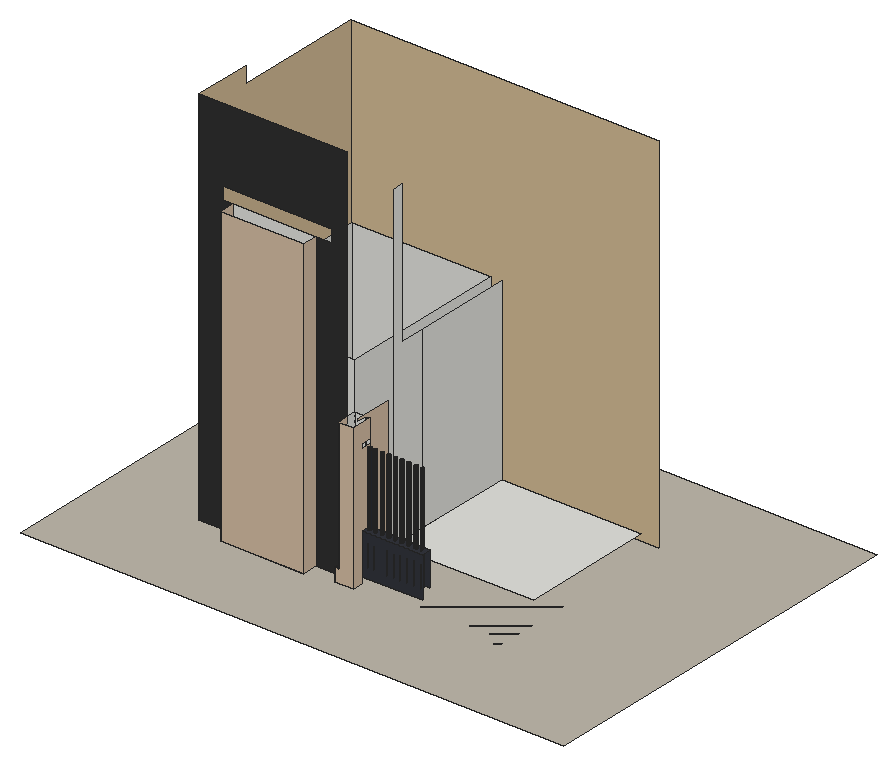
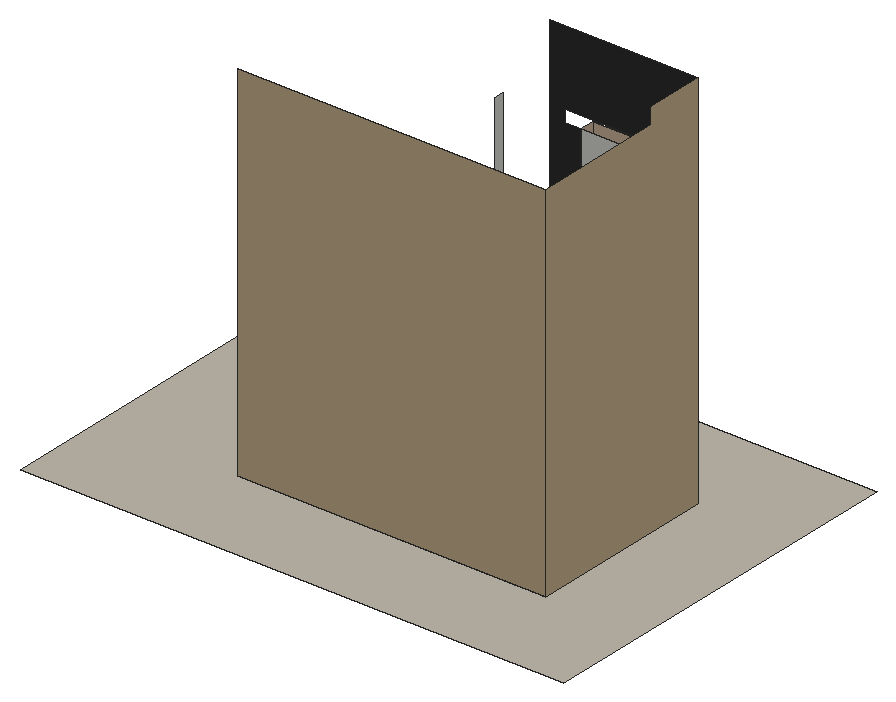
# SketchUp Ruby script. Lengths in inches.
U = 1.inch
M = Sketchup.active_model
def pt(a) = Geom::Point3d.new(a.map { |v| v * U })
def face(e, loops, mat)
  f = e.add_face(loops[0].map { |a| pt(a) })
  loops[1..].each { |l| e.add_face(l.map { |a| pt(a) }).erase! }
  f.material = f.back_material = mat if mat
  f
end
# faces: each face lists its corners as indices into pts; further lists are holes
def faces(e, pts, list, mat = nil) = list.each { |f| face(e, (f[0].is_a?(Array) ? f : [f]).map { |l| l.map { |i| pts[i] } }, mat) }
# xy, xz, yz: faces in a plane at the given z, y or x. An outline is a flat list of corners, or four numbers for a rectangle; further outlines are holes
def ring(l) = l.size == 4 ? [[l[0], l[1]], [l[2], l[1]], [l[2], l[3]], [l[0], l[3]]] : l.each_slice(2).to_a
def flat(e, list, mat, &to3) = list.each { |f| face(e, (f[0].is_a?(Array) ? f : [f]).map { |l| ring(l).map { |u, v| to3.(u, v) } }, mat) }
def xy(e, z, list, mat = nil) = flat(e, list, mat) { |x, y| [x, y, z] }
def xz(e, y, list, mat = nil) = flat(e, list, mat) { |x, z| [x, y, z] }
def yz(e, x, list, mat = nil) = flat(e, list, mat) { |y, z| [x, y, z] }
def lines(e, pts, list) = list.each { |a, b| e.add_line(pt(pts[a]), pt(pts[b])) }
# prism: a flat outline (further loops are holes) pulled along v
def prism(e, loops, v, mat = nil)
  f = face(e, loops, mat); d = Geom::Vector3d.new(v.map { |x| x * U })
  f.pushpull(f.normal.samedirection?(d) ? d.length : -d.length)
end
def box(e, o, s, mat = nil) = prism(e, [[o, [o[0] + s[0], o[1], o[2]], [o[0] + s[0], o[1] + s[1], o[2]], [o[0], o[1] + s[1], o[2]]]], [0, 0, s[2]], mat)
def at(x, y, z, deg = 0) = Geom::Transformation.translation(pt([x, y, z])) * Geom::Transformation.rotation(ORIGIN, Z_AXIS, deg.degrees)
def axes(o, x, y, z) = Geom::Transformation.new([*x, 0, *y, 0, *z, 0, *pt(o).to_a, 1])
def part(name) = M.definitions.add(name)
# library, detail: a bought-in or finely detailed component or shape, given as its bounding box
def library(name, o, s) = part(name).tap { |d| box(d.entities, o, s) }
def detail(e, o, s) = box(e.add_group.entities, o, s)
def put(e, d, t, mat = nil) = e.add_instance(d, t).tap { |i| i.material = mat if mat }
def group(e, t, mat = nil) = e.add_group.tap { |g| g.transformation = t; g.material = mat if mat }.entities
root = M.entities
M.materials.add("[Cinder Block]").color = [191, 184, 171]
M.materials.add("[Concrete Block 8x8 Gray]").color = [48, 48, 47]
M.materials.add("[Formica Beige]").color = [211, 187, 149]
M.materials.add("[Formica Laminate Dark]").color = [50, 53, 60]
M.materials.add("[Formica Laminate Light]").color = [213, 189, 164]
xy(root,0,[[87.96,59.04,144.31,69.35],[162.85,61.98,162.85,69.35,65.24,69.35,65.24,197.12,273.31,197.12,273.31,61.98,261.51,61.98,261.51,69.35,175.36,69.35,175.36,61.98]])
xy(root,0,[[[0,0,367.4375,263.4375],[87.96,59.04,144.31,69.35]]],"[Cinder Block]")
xy(root,9,[[177.5,71.93,177.24,71.96,177,72.0625,176.79,72.22,176.63,72.43,176.53,72.67,176.5,72.93,176.53,73.1875,176.63,73.43,176.79,73.63,177,73.79,177.24,73.89,177.5,73.93,177.76,73.89,178,73.79,178.21,73.63,178.37,73.43,178.46,73.1875,178.5,72.93,178.46,72.67,178.37,72.43,178.21,72.22,178,72.0625,177.76,71.96],[181.5,71.93,181.24,71.96,181,72.0625,180.79,72.22,180.63,72.43,180.53,72.67,180.5,72.93,180.53,73.1875,180.63,73.43,180.79,73.63,181,73.79,181.24,73.89,181.5,73.93,181.76,73.89,182,73.79,182.21,73.63,182.37,73.43,182.46,73.1875,182.5,72.93,182.46,72.67,182.37,72.43,182.21,72.22,182,72.0625,181.76,71.96],[186.1875,71.93,185.93,71.96,185.6875,72.0625,185.48,72.22,185.32,72.43,185.22,72.67,185.1875,72.93,185.22,73.1875,185.32,73.43,185.48,73.63,185.6875,73.79,185.93,73.89,186.1875,73.93,186.45,73.89,186.6875,73.79,186.89,73.63,187.05,73.43,187.15,73.1875,187.1875,72.93,187.15,72.67,187.05,72.43,186.89,72.22,186.6875,72.0625,186.45,71.96],[190.75,71.93,190.49,71.96,190.25,72.0625,190.04,72.22,189.88,72.43,189.78,72.67,189.75,72.93,189.78,73.1875,189.88,73.43,190.04,73.63,190.25,73.79,190.49,73.89,190.75,73.93,191.01,73.89,191.25,73.79,191.46,73.63,191.62,73.43,191.71,73.1875,191.75,72.93,191.71,72.67,191.62,72.43,191.46,72.22,191.25,72.0625,191.01,71.96],[195,71.93,194.74,71.96,194.5,72.0625,194.29,72.22,194.13,72.43,194.03,72.67,194,72.93,194.03,73.1875,194.13,73.43,194.29,73.63,194.5,73.79,194.74,73.89,195,73.93,195.26,73.89,195.5,73.79,195.71,73.63,195.87,73.43,195.96,73.1875,196,72.93,195.96,72.67,195.87,72.43,195.71,72.22,195.5,72.0625,195.26,71.96],
  [199.4375,71.93,199.18,71.96,198.9375,72.0625,198.73,72.22,198.57,72.43,198.47,72.67,198.4375,72.93,198.47,73.1875,198.57,73.43,198.73,73.63,198.9375,73.79,199.18,73.89,199.4375,73.93,199.7,73.89,199.9375,73.79,200.14,73.63,200.3,73.43,200.4,73.1875,200.4375,72.93,200.4,72.67,200.3,72.43,200.14,72.22,199.9375,72.0625,199.7,71.96],[204,71.93,203.74,71.96,203.5,72.0625,203.29,72.22,203.13,72.43,203.03,72.67,203,72.93,203.03,73.1875,203.13,73.43,203.29,73.63,203.5,73.79,203.74,73.89,204,73.93,204.26,73.89,204.5,73.79,204.71,73.63,204.87,73.43,204.96,73.1875,205,72.93,204.96,72.67,204.87,72.43,204.71,72.22,204.5,72.0625,204.26,71.96],[209.0625,71.93,208.8,71.96,208.5625,72.0625,208.35,72.22,208.2,72.43,208.1,72.67,208.0625,72.93,208.1,73.1875,208.2,73.43,208.35,73.63,208.5625,73.79,208.8,73.89,209.0625,73.93,209.32,73.89,209.5625,73.79,209.77,73.63,209.93,73.43,210.03,73.1875,210.0625,72.93,210.03,72.67,209.93,72.43,209.77,72.22,209.5625,72.0625,209.32,71.96],[71.76,75.87,165.35,190.6],[172.48,99.67,266.79,190.6]])
xy(root,9,[[162.85,61.98,165.35,69.35]],"[Formica Laminate Light]")
xy(root,32.25,[[[175.36,69.35,216.21,75.87],[177.5,71.93,177.24,71.96,177,72.0625,176.79,72.22,176.63,72.43,176.53,72.67,176.5,72.93,176.53,73.1875,176.63,73.43,176.79,73.63,177,73.79,177.24,73.89,177.5,73.93,177.76,73.89,178,73.79,178.21,73.63,178.37,73.43,178.46,73.1875,178.5,72.93,178.46,72.67,178.37,72.43,178.21,72.22,178,72.0625,177.76,71.96],[213.5,71.93,213.24,71.96,213,72.0625,212.79,72.22,212.63,72.43,212.53,72.67,212.5,72.93,212.53,73.1875,212.63,73.43,212.79,73.63,213,73.79,213.24,73.89,213.5,73.93,213.76,73.89,214,73.79,214.21,73.63,214.37,73.43,214.46,73.1875,214.5,72.93,214.46,72.67,214.37,72.43,214.21,72.22,214,72.0625,213.76,71.96],[181.5,71.93,181.24,71.96,181,72.0625,180.79,72.22,180.63,72.43,180.53,72.67,180.5,72.93,180.53,73.1875,180.63,73.43,180.79,73.63,181,73.79,181.24,73.89,181.5,73.93,181.76,73.89,182,73.79,182.21,73.63,182.37,73.43,182.46,73.1875,182.5,72.93,182.46,72.67,182.37,72.43,182.21,72.22,182,72.0625,181.76,71.96],[209.0625,71.93,208.8,71.96,208.5625,72.0625,208.35,72.22,208.2,72.43,208.1,72.67,208.0625,72.93,208.1,73.1875,208.2,73.43,208.35,73.63,208.5625,73.79,208.8,73.89,209.0625,73.93,209.32,73.89,209.5625,73.79,209.77,73.63,209.93,73.43,210.03,73.1875,210.0625,72.93,210.03,72.67,209.93,72.43,209.77,72.22,209.5625,72.0625,209.32,71.96],[186.1875,71.93,185.93,71.96,185.6875,72.0625,185.48,72.22,185.32,72.43,185.22,72.67,185.1875,72.93,185.22,73.1875,185.32,73.43,185.48,73.63,185.6875,73.79,185.93,73.89,186.1875,73.93,186.45,73.89,186.6875,73.79,186.89,73.63,187.05,73.43,187.15,73.1875,187.1875,72.93,187.15,72.67,187.05,72.43,186.89,72.22,186.6875,72.0625,186.45,71.96],[204,71.93,203.74,71.96,203.5,72.0625,203.29,72.22,203.13,72.43,203.03,72.67,203,72.93,203.03,73.1875,203.13,73.43,203.29,73.63,203.5,73.79,203.74,73.89,204,73.93,204.26,73.89,204.5,73.79,204.71,73.63,204.87,73.43,204.96,73.1875,205,72.93,204.96,72.67,204.87,72.43,204.71,72.22,204.5,72.0625,204.26,71.96],[190.75,71.93,190.49,71.96,190.25,72.0625,190.04,72.22,189.88,72.43,189.78,72.67,189.75,72.93,189.78,73.1875,189.88,73.43,190.04,73.63,190.25,73.79,190.49,73.89,190.75,73.93,191.01,73.89,191.25,73.79,191.46,73.63,191.62,73.43,191.71,73.1875,191.75,72.93,191.71,72.67,191.62,72.43,191.46,72.22,191.25,72.0625,191.01,71.96],[199.4375,71.93,199.18,71.96,198.9375,72.0625,198.73,72.22,198.57,72.43,198.47,72.67,198.4375,72.93,198.47,73.1875,198.57,73.43,198.73,73.63,198.9375,73.79,199.18,73.89,199.4375,73.93,199.7,73.89,199.9375,73.79,200.14,73.63,200.3,73.43,200.4,73.1875,200.4375,72.93,200.4,72.67,200.3,72.43,200.14,72.22,199.9375,72.0625,199.7,71.96],[195,71.93,194.74,71.96,194.5,72.0625,194.29,72.22,194.13,72.43,194.03,72.67,194,72.93,194.03,73.1875,194.13,73.43,194.29,73.63,194.5,73.79,194.74,73.89,195,73.93,195.26,73.89,195.5,73.79,195.71,73.63,195.87,73.43,195.96,73.1875,196,72.93,195.96,72.67,195.87,72.43,195.71,72.22,195.5,72.0625,195.26,71.96]]],"[Formica Laminate Dark]")
xz(root,59.04,[[87.96,0,144.31,199.15]],"[Formica Laminate Light]")
xz(root,61.98,[[162.85,0,175.36,0,175.36,97.5,165.35,97.5,165.35,9,162.85,9]],"[Formica Laminate Light]")
xz(root,69.35,[[87.96,0,144.31,199.15]])
xz(root,69.35,[[65.24,0,87.96,0,87.96,199.15,81.08,199.15,81.08,207.68,154.75,207.68,154.75,199.15,144.31,199.15,144.31,0,162.85,0,162.85,9,165.35,9,165.35,257.76,65.24,257.76]],"[Concrete Block 8x8 Gray]")
xz(root,69.35,[[175.36,4.5,216.21,32.25]],"[Formica Laminate Dark]")
xz(root,75.87,[[71.76,9,165.35,129],[165.35,9,172.48,97.5],[172.48,9,175.36,97.5]])
xz(root,75.87,[[175.36,9,216.21,32.25]],"[Formica Laminate Dark]")
xz(root,190.6,[[71.76,9,165.35,129]])
xz(root,197.12,[[65.24,0,273.31,246.5]],"[Formica Beige]")
yz(root,65.24,[[69.35,0,69.35,257.76,108.74,257.76,108.74,246.5,197.12,246.5,197.12,0]],"[Formica Beige]")
yz(root,71.76,[[75.87,9,190.6,129]])
yz(root,87.96,[[59.04,0,69.35,199.15]],"[Formica Laminate Light]")
yz(root,144.31,[[59.04,0,69.35,199.15]],"[Formica Laminate Light]")
yz(root,162.85,[[61.98,0,69.35,9]],"[Formica Laminate Light]")
yz(root,165.35,[[69.35,9,75.87,97.5],[75.87,9,190.6,129]])
yz(root,165.35,[[61.98,9,69.35,97.5]],"[Formica Laminate Light]")
yz(root,172.48,[[99.67,9,123.48,9,123.48,129,106.73,129,106.73,224.375,99.67,224.375],[123.48,9,190.6,129]])
yz(root,172.48,[[75.87,9,94.48,9,94.48,98.95,69.35,98.95,69.35,97.5,75.87,97.5]],"[Formica Laminate Light]")
yz(root,175.36,[[61.98,0,69.35,0,69.35,32.25,75.87,32.25,75.87,81.84,69.35,81.84,69.35,84.9,75.87,84.9,75.87,97.5,61.98,97.5]],"[Formica Laminate Light]")
p = [[177.24,71.96,9],[177.5,71.93,9],[177.5,71.93,32.25],[177.24,71.96,32.25],[177.76,71.96,9],[177.76,71.96,32.25],
  [181.24,71.96,9],[181.5,71.93,9],[181.5,71.93,32.25],[181.24,71.96,32.25],[181.76,71.96,9],[181.76,71.96,32.25],
  [185.93,71.96,9],[186.1875,71.93,9],[186.1875,71.93,32.25],[185.93,71.96,32.25],[186.45,71.96,9],[186.45,71.96,32.25],
  [190.49,71.96,9],[190.75,71.93,9],[190.75,71.93,32.25],[190.49,71.96,32.25],[191.01,71.96,9],[191.01,71.96,32.25],
  [194.74,71.96,9],[195,71.93,9],[195,71.93,32.25],[194.74,71.96,32.25],[195.26,71.96,9],[195.26,71.96,32.25],
  [199.18,71.96,9],[199.4375,71.93,9],[199.4375,71.93,32.25],[199.18,71.96,32.25],[199.7,71.96,9],[199.7,71.96,32.25],
  [203.74,71.96,9],[204,71.93,9],[204,71.93,32.25],[203.74,71.96,32.25],[204.26,71.96,9],[204.26,71.96,32.25],
  [208.8,71.96,9],[209.0625,71.93,9],[209.0625,71.93,32.25],[208.8,71.96,32.25],[209.32,71.96,9],[209.32,71.96,32.25],
  [213.24,71.96,9],[213.5,71.93,9],[213.5,71.93,32.25],[213.24,71.96,32.25],[177,72.0625,9],[177,72.0625,32.25],
  [178,72.0625,9],[178,72.0625,32.25],[181,72.0625,9],[181,72.0625,32.25],[182,72.0625,9],[182,72.0625,32.25],
  [185.6875,72.0625,9],[185.6875,72.0625,32.25],[186.6875,72.0625,9],[186.6875,72.0625,32.25],[190.25,72.0625,9],[190.25,72.0625,32.25],
  [191.25,72.0625,9],[191.25,72.0625,32.25],[194.5,72.0625,9],[194.5,72.0625,32.25],[195.5,72.0625,9],[195.5,72.0625,32.25],
  [198.9375,72.0625,9],[198.9375,72.0625,32.25],[199.9375,72.0625,9],[199.9375,72.0625,32.25],[203.5,72.0625,9],[203.5,72.0625,32.25],
  [204.5,72.0625,9],[204.5,72.0625,32.25],[208.5625,72.0625,9],[208.5625,72.0625,32.25],[209.5625,72.0625,9],[209.5625,72.0625,32.25],
  [213,72.0625,9],[213,72.0625,32.25],[176.79,72.22,9],[176.79,72.22,32.25],[178.21,72.22,9],[178.21,72.22,32.25],
  [180.79,72.22,9],[180.79,72.22,32.25],[182.21,72.22,9],[182.21,72.22,32.25],[185.48,72.22,9],[185.48,72.22,32.25],
  [186.89,72.22,9],[186.89,72.22,32.25],[190.04,72.22,9],[190.04,72.22,32.25],[191.46,72.22,9],[191.46,72.22,32.25],
  [194.29,72.22,9],[194.29,72.22,32.25],[195.71,72.22,9],[195.71,72.22,32.25],[198.73,72.22,9],[198.73,72.22,32.25],
  [200.14,72.22,9],[200.14,72.22,32.25],[203.29,72.22,9],[203.29,72.22,32.25],[204.71,72.22,9],[204.71,72.22,32.25],
  [208.35,72.22,9],[208.35,72.22,32.25],[209.77,72.22,9],[209.77,72.22,32.25],[212.79,72.22,9],[212.79,72.22,32.25],
  [176.63,72.43,9],[176.63,72.43,32.25],[178.37,72.43,9],[178.37,72.43,32.25],[180.63,72.43,9],[180.63,72.43,32.25],
  [182.37,72.43,9],[182.37,72.43,32.25],[185.32,72.43,9],[185.32,72.43,32.25],[187.05,72.43,9],[187.05,72.43,32.25],
  [189.88,72.43,9],[189.88,72.43,32.25],[191.62,72.43,9],[191.62,72.43,32.25],[194.13,72.43,9],[194.13,72.43,32.25],
  [195.87,72.43,9],[195.87,72.43,32.25],[198.57,72.43,9],[198.57,72.43,32.25],[200.3,72.43,9],[200.3,72.43,32.25],
  [203.13,72.43,9],[203.13,72.43,32.25],[204.87,72.43,9],[204.87,72.43,32.25],[208.2,72.43,9],[208.2,72.43,32.25],
  [209.93,72.43,9],[209.93,72.43,32.25],[212.63,72.43,9],[212.63,72.43,32.25],[176.53,72.67,9],[176.53,72.67,32.25],
  [178.46,72.67,9],[178.46,72.67,32.25],[180.53,72.67,9],[180.53,72.67,32.25],[182.46,72.67,9],[182.46,72.67,32.25],
  [185.22,72.67,9],[185.22,72.67,32.25],[187.15,72.67,9],[187.15,72.67,32.25],[189.78,72.67,9],[189.78,72.67,32.25],
  [191.71,72.67,9],[191.71,72.67,32.25],[194.03,72.67,9],[194.03,72.67,32.25],[195.96,72.67,9],[195.96,72.67,32.25],
  [198.47,72.67,9],[198.47,72.67,32.25],[200.4,72.67,9],[200.4,72.67,32.25],[203.03,72.67,9],[203.03,72.67,32.25],
  [204.96,72.67,9],[204.96,72.67,32.25],[208.1,72.67,9],[208.1,72.67,32.25],[210.03,72.67,9],[210.03,72.67,32.25],
  [212.53,72.67,9],[212.53,72.67,32.25],[176.5,72.93,9],[176.5,72.93,32.25],[178.5,72.93,9],[178.5,72.93,32.25],
  [180.5,72.93,9],[180.5,72.93,32.25],[182.5,72.93,9],[182.5,72.93,32.25],[185.1875,72.93,9],[185.1875,72.93,32.25],
  [187.1875,72.93,9],[187.1875,72.93,32.25],[189.75,72.93,9],[189.75,72.93,32.25],[191.75,72.93,9],[191.75,72.93,32.25],
  [194,72.93,9],[194,72.93,32.25],[196,72.93,9],[196,72.93,32.25],[198.4375,72.93,9],[198.4375,72.93,32.25],
  [200.4375,72.93,9],[200.4375,72.93,32.25],[203,72.93,9],[203,72.93,32.25],[205,72.93,9],[205,72.93,32.25],
  [208.0625,72.93,9],[208.0625,72.93,32.25],[210.0625,72.93,9],[210.0625,72.93,32.25],[212.5,72.93,9],[212.5,72.93,32.25],
  [176.53,73.1875,9],[176.53,73.1875,32.25],[178.46,73.1875,9],[178.46,73.1875,32.25],[180.53,73.1875,9],[180.53,73.1875,32.25],
  [182.46,73.1875,9],[182.46,73.1875,32.25],[185.22,73.1875,9],[185.22,73.1875,32.25],[187.15,73.1875,9],[187.15,73.1875,32.25],
  [189.78,73.1875,9],[189.78,73.1875,32.25],[191.71,73.1875,9],[191.71,73.1875,32.25],[194.03,73.1875,9],[194.03,73.1875,32.25],
  [195.96,73.1875,9],[195.96,73.1875,32.25],[198.47,73.1875,9],[198.47,73.1875,32.25],[200.4,73.1875,9],[200.4,73.1875,32.25],
  [203.03,73.1875,9],[203.03,73.1875,32.25],[204.96,73.1875,9],[204.96,73.1875,32.25],[208.1,73.1875,9],[208.1,73.1875,32.25],
  [210.03,73.1875,9],[210.03,73.1875,32.25],[212.53,73.1875,9],[212.53,73.1875,32.25],[176.63,73.43,9],[176.63,73.43,32.25],
  [178.37,73.43,9],[178.37,73.43,32.25],[180.63,73.43,9],[180.63,73.43,32.25],[182.37,73.43,9],[182.37,73.43,32.25],
  [185.32,73.43,9],[185.32,73.43,32.25],[187.05,73.43,9],[187.05,73.43,32.25],[189.88,73.43,9],[189.88,73.43,32.25],
  [191.62,73.43,9],[191.62,73.43,32.25],[194.13,73.43,9],[194.13,73.43,32.25],[195.87,73.43,9],[195.87,73.43,32.25],
  [198.57,73.43,9],[198.57,73.43,32.25],[200.3,73.43,9],[200.3,73.43,32.25],[203.13,73.43,9],[203.13,73.43,32.25],
  [204.87,73.43,9],[204.87,73.43,32.25],[208.2,73.43,9],[208.2,73.43,32.25],[209.93,73.43,9],[209.93,73.43,32.25],
  [212.63,73.43,9],[212.63,73.43,32.25],[176.79,73.63,9],[176.79,73.63,32.25],[178.21,73.63,9],[178.21,73.63,32.25],
  [180.79,73.63,9],[180.79,73.63,32.25],[182.21,73.63,9],[182.21,73.63,32.25],[185.48,73.63,9],[185.48,73.63,32.25],
  [186.89,73.63,9],[186.89,73.63,32.25],[190.04,73.63,9],[190.04,73.63,32.25],[191.46,73.63,9],[191.46,73.63,32.25],
  [194.29,73.63,9],[194.29,73.63,32.25],[195.71,73.63,9],[195.71,73.63,32.25],[198.73,73.63,9],[198.73,73.63,32.25],
  [200.14,73.63,9],[200.14,73.63,32.25],[203.29,73.63,9],[203.29,73.63,32.25],[204.71,73.63,9],[204.71,73.63,32.25],
  [208.35,73.63,9],[208.35,73.63,32.25],[209.77,73.63,9],[209.77,73.63,32.25],[212.79,73.63,9],[212.79,73.63,32.25],
  [177,73.79,9],[177,73.79,32.25],[178,73.79,9],[178,73.79,32.25],[181,73.79,9],[181,73.79,32.25],
  [182,73.79,9],[182,73.79,32.25],[185.6875,73.79,9],[185.6875,73.79,32.25],[186.6875,73.79,9],[186.6875,73.79,32.25],
  [190.25,73.79,9],[190.25,73.79,32.25],[191.25,73.79,9],[191.25,73.79,32.25],[194.5,73.79,9],[194.5,73.79,32.25],
  [195.5,73.79,9],[195.5,73.79,32.25],[198.9375,73.79,9],[198.9375,73.79,32.25],[199.9375,73.79,9],[199.9375,73.79,32.25],
  [203.5,73.79,9],[203.5,73.79,32.25],[204.5,73.79,9],[204.5,73.79,32.25],[208.5625,73.79,9],[208.5625,73.79,32.25],
  [209.5625,73.79,9],[209.5625,73.79,32.25],[213,73.79,9],[213,73.79,32.25],[177.24,73.89,9],[177.24,73.89,32.25],
  [177.76,73.89,9],[177.76,73.89,32.25],[181.24,73.89,9],[181.24,73.89,32.25],[181.76,73.89,9],[181.76,73.89,32.25],
  [185.93,73.89,9],[185.93,73.89,32.25],[186.45,73.89,9],[186.45,73.89,32.25],[190.49,73.89,9],[190.49,73.89,32.25],
  [191.01,73.89,9],[191.01,73.89,32.25],[194.74,73.89,9],[194.74,73.89,32.25],[195.26,73.89,9],[195.26,73.89,32.25],
  [199.18,73.89,9],[199.18,73.89,32.25],[199.7,73.89,9],[199.7,73.89,32.25],[203.74,73.89,9],[203.74,73.89,32.25],
  [204.26,73.89,9],[204.26,73.89,32.25],[208.8,73.89,9],[208.8,73.89,32.25],[209.32,73.89,9],[209.32,73.89,32.25],
  [213.24,73.89,9],[213.24,73.89,32.25],[177.5,73.93,9],[177.5,73.93,32.25],[181.5,73.93,9],[181.5,73.93,32.25],
  [186.1875,73.93,9],[186.1875,73.93,32.25],[190.75,73.93,9],[190.75,73.93,32.25],[195,73.93,9],[195,73.93,32.25],
  [199.4375,73.93,9],[199.4375,73.93,32.25],[204,73.93,9],[204,73.93,32.25],[209.0625,73.93,9],[209.0625,73.93,32.25],
  [213.5,73.93,9],[213.5,73.93,32.25],[177.24,71.96,81.84],[177.5,71.93,81.84],[177.76,71.96,81.84],[181.24,71.96,81.84],
  [181.5,71.93,81.84],[181.76,71.96,81.84],[185.93,71.96,81.84],[186.1875,71.93,81.84],[186.45,71.96,81.84],[190.49,71.96,81.84],
  [190.75,71.93,81.84],[191.01,71.96,81.84],[194.74,71.96,81.84],[195,71.93,81.84],[195.26,71.96,81.84],[199.18,71.96,81.84],
  [199.4375,71.93,81.84],[199.7,71.96,81.84],[203.74,71.96,81.84],[204,71.93,81.84],[204.26,71.96,81.84],[208.8,71.96,81.84],
  [209.0625,71.93,81.84],[209.32,71.96,81.84],[177,72.0625,81.84],[178,72.0625,81.84],[181,72.0625,81.84],[182,72.0625,81.84],
  [185.6875,72.0625,81.84],[186.6875,72.0625,81.84],[190.25,72.0625,81.84],[191.25,72.0625,81.84],[194.5,72.0625,81.84],[195.5,72.0625,81.84],
  [198.9375,72.0625,81.84],[199.9375,72.0625,81.84],[203.5,72.0625,81.84],[204.5,72.0625,81.84],[208.5625,72.0625,81.84],[209.5625,72.0625,81.84],
  [213,72.0625,81.84],[213.24,71.96,81.84],[176.79,72.22,81.84],[178.21,72.22,81.84],[180.79,72.22,81.84],[182.21,72.22,81.84],
  [185.48,72.22,81.84],[186.89,72.22,81.84],[190.04,72.22,81.84],[191.46,72.22,81.84],[194.29,72.22,81.84],[195.71,72.22,81.84],
  [198.73,72.22,81.84],[200.14,72.22,81.84],[203.29,72.22,81.84],[204.71,72.22,81.84],[208.35,72.22,81.84],[209.77,72.22,81.84],
  [212.79,72.22,81.84],[176.63,72.43,81.84],[178.37,72.43,81.84],[180.63,72.43,81.84],[182.37,72.43,81.84],[185.32,72.43,81.84],
  [187.05,72.43,81.84],[189.88,72.43,81.84],[191.62,72.43,81.84],[194.13,72.43,81.84],[195.87,72.43,81.84],[198.57,72.43,81.84],
  [200.3,72.43,81.84],[203.13,72.43,81.84],[204.87,72.43,81.84],[208.2,72.43,81.84],[209.93,72.43,81.84],[212.63,72.43,81.84],
  [176.53,72.67,81.84],[178.46,72.67,81.84],[180.53,72.67,81.84],[182.46,72.67,81.84],[185.22,72.67,81.84],[187.15,72.67,81.84],
  [189.78,72.67,81.84],[191.71,72.67,81.84],[194.03,72.67,81.84],[195.96,72.67,81.84],[198.47,72.67,81.84],[200.4,72.67,81.84],
  [203.03,72.67,81.84],[204.96,72.67,81.84],[208.1,72.67,81.84],[210.03,72.67,81.84],[212.53,72.67,81.84],[176.5,72.93,81.84],
  [178.5,72.93,81.84],[180.5,72.93,81.84],[182.5,72.93,81.84],[185.1875,72.93,81.84],[187.1875,72.93,81.84],[189.75,72.93,81.84],
  [191.75,72.93,81.84],[194,72.93,81.84],[196,72.93,81.84],[198.4375,72.93,81.84],[200.4375,72.93,81.84],[203,72.93,81.84],
  [205,72.93,81.84],[208.0625,72.93,81.84],[210.0625,72.93,81.84],[212.5,72.93,81.84],[176.53,73.1875,81.84],[178.46,73.1875,81.84],
  [180.53,73.1875,81.84],[182.46,73.1875,81.84],[185.22,73.1875,81.84],[187.15,73.1875,81.84],[189.78,73.1875,81.84],[191.71,73.1875,81.84],
  [194.03,73.1875,81.84],[195.96,73.1875,81.84],[198.47,73.1875,81.84],[200.4,73.1875,81.84],[203.03,73.1875,81.84],[204.96,73.1875,81.84],
  [208.1,73.1875,81.84],[210.03,73.1875,81.84],[212.53,73.1875,81.84],[176.63,73.43,81.84],[178.37,73.43,81.84],[180.63,73.43,81.84],
  [182.37,73.43,81.84],[185.32,73.43,81.84],[187.05,73.43,81.84],[189.88,73.43,81.84],[191.62,73.43,81.84],[194.13,73.43,81.84],
  [195.87,73.43,81.84],[198.57,73.43,81.84],[200.3,73.43,81.84],[203.13,73.43,81.84],[204.87,73.43,81.84],[208.2,73.43,81.84],
  [209.93,73.43,81.84],[212.63,73.43,81.84],[176.79,73.63,81.84],[178.21,73.63,81.84],[180.79,73.63,81.84],[182.21,73.63,81.84],
  [185.48,73.63,81.84],[186.89,73.63,81.84],[190.04,73.63,81.84],[191.46,73.63,81.84],[194.29,73.63,81.84],[195.71,73.63,81.84],
  [198.73,73.63,81.84],[200.14,73.63,81.84],[203.29,73.63,81.84],[204.71,73.63,81.84],[208.35,73.63,81.84],[209.77,73.63,81.84],
  [212.79,73.63,81.84],[177,73.79,81.84],[178,73.79,81.84],[181,73.79,81.84],[182,73.79,81.84],[185.6875,73.79,81.84],
  [186.6875,73.79,81.84],[190.25,73.79,81.84],[191.25,73.79,81.84],[194.5,73.79,81.84],[195.5,73.79,81.84],[198.9375,73.79,81.84],
  [199.9375,73.79,81.84],[203.5,73.79,81.84],[204.5,73.79,81.84],[208.5625,73.79,81.84],[209.5625,73.79,81.84],[213,73.79,81.84],
  [177.24,73.89,81.84],[177.76,73.89,81.84],[181.24,73.89,81.84],[181.76,73.89,81.84],[185.93,73.89,81.84],[186.45,73.89,81.84],
  [190.49,73.89,81.84],[191.01,73.89,81.84],[194.74,73.89,81.84],[195.26,73.89,81.84],[199.18,73.89,81.84],[199.7,73.89,81.84],
  [203.74,73.89,81.84],[204.26,73.89,81.84],[208.8,73.89,81.84],[209.32,73.89,81.84],[213.24,73.89,81.84],[177.5,73.93,81.84],
  [181.5,73.93,81.84],[186.1875,73.93,81.84],[190.75,73.93,81.84],[195,73.93,81.84],[199.4375,73.93,81.84],[204,73.93,81.84],
  [209.0625,73.93,81.84]]
faces(root,p,[[0,1,2,3],[1,4,5,2],[6,7,8,9],[7,10,11,8],[12,13,14,15],[13,16,17,14],[18,19,20,21],[19,22,23,20],
  [24,25,26,27],[25,28,29,26],[30,31,32,33],[31,34,35,32],[36,37,38,39],[37,40,41,38],[42,43,44,45],[43,46,47,44],
  [48,49,50,51],[52,0,3,53],[4,54,55,5],[56,6,9,57],[10,58,59,11],[60,12,15,61],[16,62,63,17],[64,18,21,65],
  [22,66,67,23],[68,24,27,69],[28,70,71,29],[72,30,33,73],[34,74,75,35],[76,36,39,77],[40,78,79,41],[80,42,45,81],
  [46,82,83,47],[84,48,51,85],[86,52,53,87],[54,88,89,55],[90,56,57,91],[58,92,93,59],[94,60,61,95],[62,96,97,63],
  [98,64,65,99],[66,100,101,67],[102,68,69,103],[70,104,105,71],[106,72,73,107],[74,108,109,75],[110,76,77,111],[78,112,113,79],
  [114,80,81,115],[82,116,117,83],[118,84,85,119],[120,86,87,121],[88,122,123,89],[124,90,91,125],[92,126,127,93],[128,94,95,129],
  [96,130,131,97],[132,98,99,133],[100,134,135,101],[136,102,103,137],[104,138,139,105],[140,106,107,141],[108,142,143,109],[144,110,111,145],
  [112,146,147,113],[148,114,115,149],[116,150,151,117],[152,118,119,153],[154,120,121,155],[122,156,157,123],[158,124,125,159],[126,160,161,127],
  [162,128,129,163],[130,164,165,131],[166,132,133,167],[134,168,169,135],[170,136,137,171],[138,172,173,139],[174,140,141,175],[142,176,177,143],
  [178,144,145,179],[146,180,181,147],[182,148,149,183],[150,184,185,151],[186,152,153,187],[188,154,155,189],[156,190,191,157],[192,158,159,193],
  [160,194,195,161],[196,162,163,197],[164,198,199,165],[200,166,167,201],[168,202,203,169],[204,170,171,205],[172,206,207,173],[208,174,175,209],
  [176,210,211,177],[212,178,179,213],[180,214,215,181],[216,182,183,217],[184,218,219,185],[220,186,187,221],[222,188,189,223],[190,224,225,191],
  [226,192,193,227],[194,228,229,195],[230,196,197,231],[198,232,233,199],[234,200,201,235],[202,236,237,203],[238,204,205,239],[206,240,241,207],
  [242,208,209,243],[210,244,245,211],[246,212,213,247],[214,248,249,215],[250,216,217,251],[218,252,253,219],[254,220,221,255],[256,222,223,257],
  [224,258,259,225],[260,226,227,261],[228,262,263,229],[264,230,231,265],[232,266,267,233],[268,234,235,269],[236,270,271,237],[272,238,239,273],
  [240,274,275,241],[276,242,243,277],[244,278,279,245],[280,246,247,281],[248,282,283,249],[284,250,251,285],[252,286,287,253],[288,254,255,289],
  [290,256,257,291],[258,292,293,259],[294,260,261,295],[262,296,297,263],[298,264,265,299],[266,300,301,267],[302,268,269,303],[270,304,305,271],
  [306,272,273,307],[274,308,309,275],[310,276,277,311],[278,312,313,279],[314,280,281,315],[282,316,317,283],[318,284,285,319],[286,320,321,287],
  [322,288,289,323],[324,290,291,325],[292,326,327,293],[328,294,295,329],[296,330,331,297],[332,298,299,333],[300,334,335,301],[336,302,303,337],
  [304,338,339,305],[340,306,307,341],[308,342,343,309],[344,310,311,345],[312,346,347,313],[348,314,315,349],[316,350,351,317],[352,318,319,353],
  [320,354,355,321],[356,322,323,357],[358,324,325,359],[326,360,361,327],[362,328,329,363],[330,364,365,331],[366,332,333,367],[334,368,369,335],
  [370,336,337,371],[338,372,373,339],[374,340,341,375],[342,376,377,343],[378,344,345,379],[346,380,381,347],[382,348,349,383],[350,384,385,351],
  [386,352,353,387],[354,388,389,355],[390,356,357,391],[392,358,359,393],[360,392,393,361],[394,362,363,395],[364,394,395,365],[396,366,367,397],
  [368,396,397,369],[398,370,371,399],[372,398,399,373],[400,374,375,401],[376,400,401,377],[402,378,379,403],[380,402,403,381],[404,382,383,405],
  [384,404,405,385],[406,386,387,407],[388,406,407,389],[408,390,391,409],[410,3,2,411],[411,2,5,412],[413,9,8,414],[414,8,11,415],
  [416,15,14,417],[417,14,17,418],[419,21,20,420],[420,20,23,421],[422,27,26,423],[423,26,29,424],[425,33,32,426],[426,32,35,427],
  [428,39,38,429],[429,38,41,430],[431,45,44,432],[432,44,47,433],[434,53,3,410],[412,5,55,435],[436,57,9,413],[415,11,59,437],
  [438,61,15,416],[418,17,63,439],[440,65,21,419],[421,23,67,441],[442,69,27,422],[424,29,71,443],[444,73,33,425],[427,35,75,445],
  [446,77,39,428],[430,41,79,447],[448,81,45,431],[433,47,83,449],[450,85,51,451],[452,87,53,434],[435,55,89,453],[454,91,57,436],
  [437,59,93,455],[456,95,61,438],[439,63,97,457],[458,99,65,440],[441,67,101,459],[460,103,69,442],[443,71,105,461],[462,107,73,444],
  [445,75,109,463],[464,111,77,446],[447,79,113,465],[466,115,81,448],[449,83,117,467],[468,119,85,450],[469,121,87,452],[453,89,123,470],
  [471,125,91,454],[455,93,127,472],[473,129,95,456],[457,97,131,474],[475,133,99,458],[459,101,135,476],[477,137,103,460],[461,105,139,478],
  [479,141,107,462],[463,109,143,480],[481,145,111,464],[465,113,147,482],[483,149,115,466],[467,117,151,484],[485,153,119,468],[486,155,121,469],
  [470,123,157,487],[488,159,125,471],[472,127,161,489],[490,163,129,473],[474,131,165,491],[492,167,133,475],[476,135,169,493],[494,171,137,477],
  [478,139,173,495],[496,175,141,479],[480,143,177,497],[498,179,145,481],[482,147,181,499],[500,183,149,483],[484,151,185,501],[502,187,153,485],
  [503,189,155,486],[487,157,191,504],[505,193,159,488],[489,161,195,506],[507,197,163,490],[491,165,199,508],[509,201,167,492],[493,169,203,510],
  [511,205,171,494],[495,173,207,512],[513,209,175,496],[497,177,211,514],[515,213,179,498],[499,181,215,516],[517,217,183,500],[501,185,219,518],
  [519,221,187,502],[520,223,189,503],[504,191,225,521],[522,227,193,505],[506,195,229,523],[524,231,197,507],[508,199,233,525],[526,235,201,509],
  [510,203,237,527],[528,239,205,511],[512,207,241,529],[530,243,209,513],[514,211,245,531],[532,247,213,515],[516,215,249,533],[534,251,217,517],
  [518,219,253,535],[536,255,221,519],[537,257,223,520],[521,225,259,538],[539,261,227,522],[523,229,263,540],[541,265,231,524],[525,233,267,542],
  [543,269,235,526],[527,237,271,544],[545,273,239,528],[529,241,275,546],[547,277,243,530],[531,245,279,548],[549,281,247,532],[533,249,283,550],
  [551,285,251,534],[535,253,287,552],[553,289,255,536],[554,291,257,537],[538,259,293,555],[556,295,261,539],[540,263,297,557],[558,299,265,541],
  [542,267,301,559],[560,303,269,543],[544,271,305,561],[562,307,273,545],[546,275,309,563],[564,311,277,547],[548,279,313,565],[566,315,281,549],
  [550,283,317,567],[568,319,285,551],[552,287,321,569],[570,323,289,553],[571,325,291,554],[555,293,327,572],[573,329,295,556],[557,297,331,574],
  [575,333,299,558],[559,301,335,576],[577,337,303,560],[561,305,339,578],[579,341,307,562],[563,309,343,580],[581,345,311,564],[565,313,347,582],
  [583,349,315,566],[567,317,351,584],[585,353,319,568],[569,321,355,586],[587,357,323,570],[588,359,325,571],[572,327,361,589],[590,363,329,573],
  [574,331,365,591],[592,367,333,575],[576,335,369,593],[594,371,337,577],[578,339,373,595],[596,375,341,579],[580,343,377,597],[598,379,345,581],
  [582,347,381,599],[600,383,349,583],[584,351,385,601],[602,387,353,585],[586,355,389,603],[604,391,357,587],[605,393,359,588],[589,361,393,605],
  [606,395,363,590],[591,365,395,606],[607,397,367,592],[593,369,397,607],[608,399,371,594],[595,373,399,608],[609,401,375,596],[597,377,401,609],
  [610,403,379,598],[599,381,403,610],[611,405,383,600],[601,385,405,611],[612,407,387,602],[603,389,407,612]],"[Formica Laminate Dark]")
